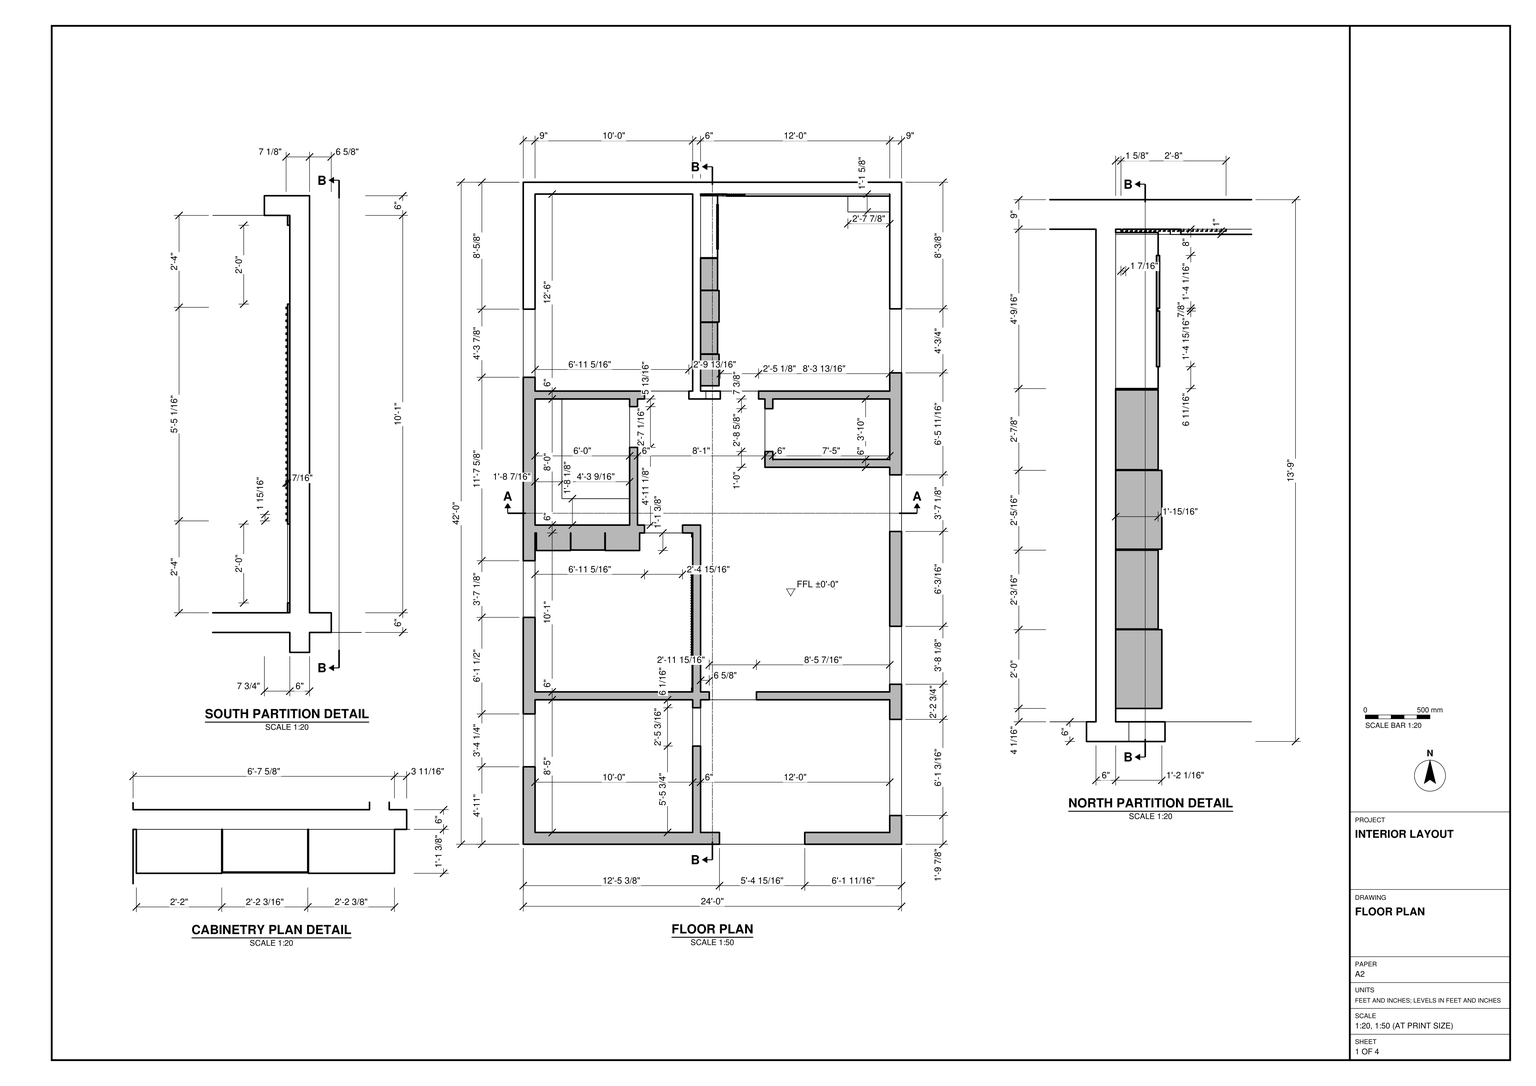
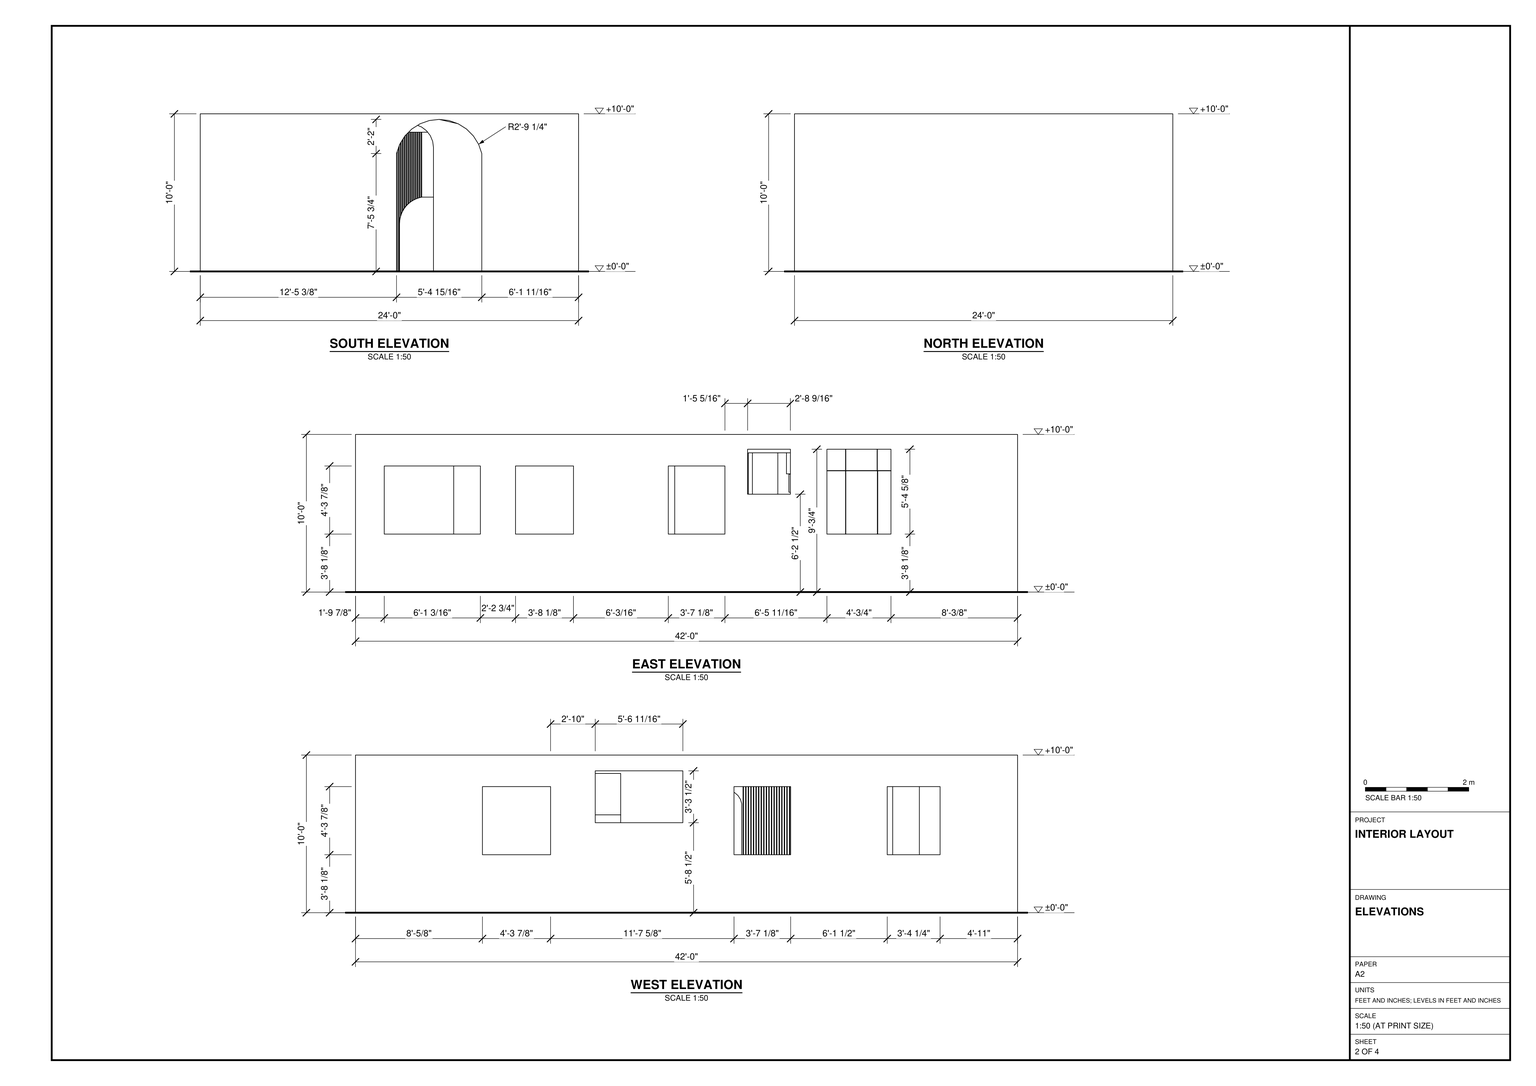
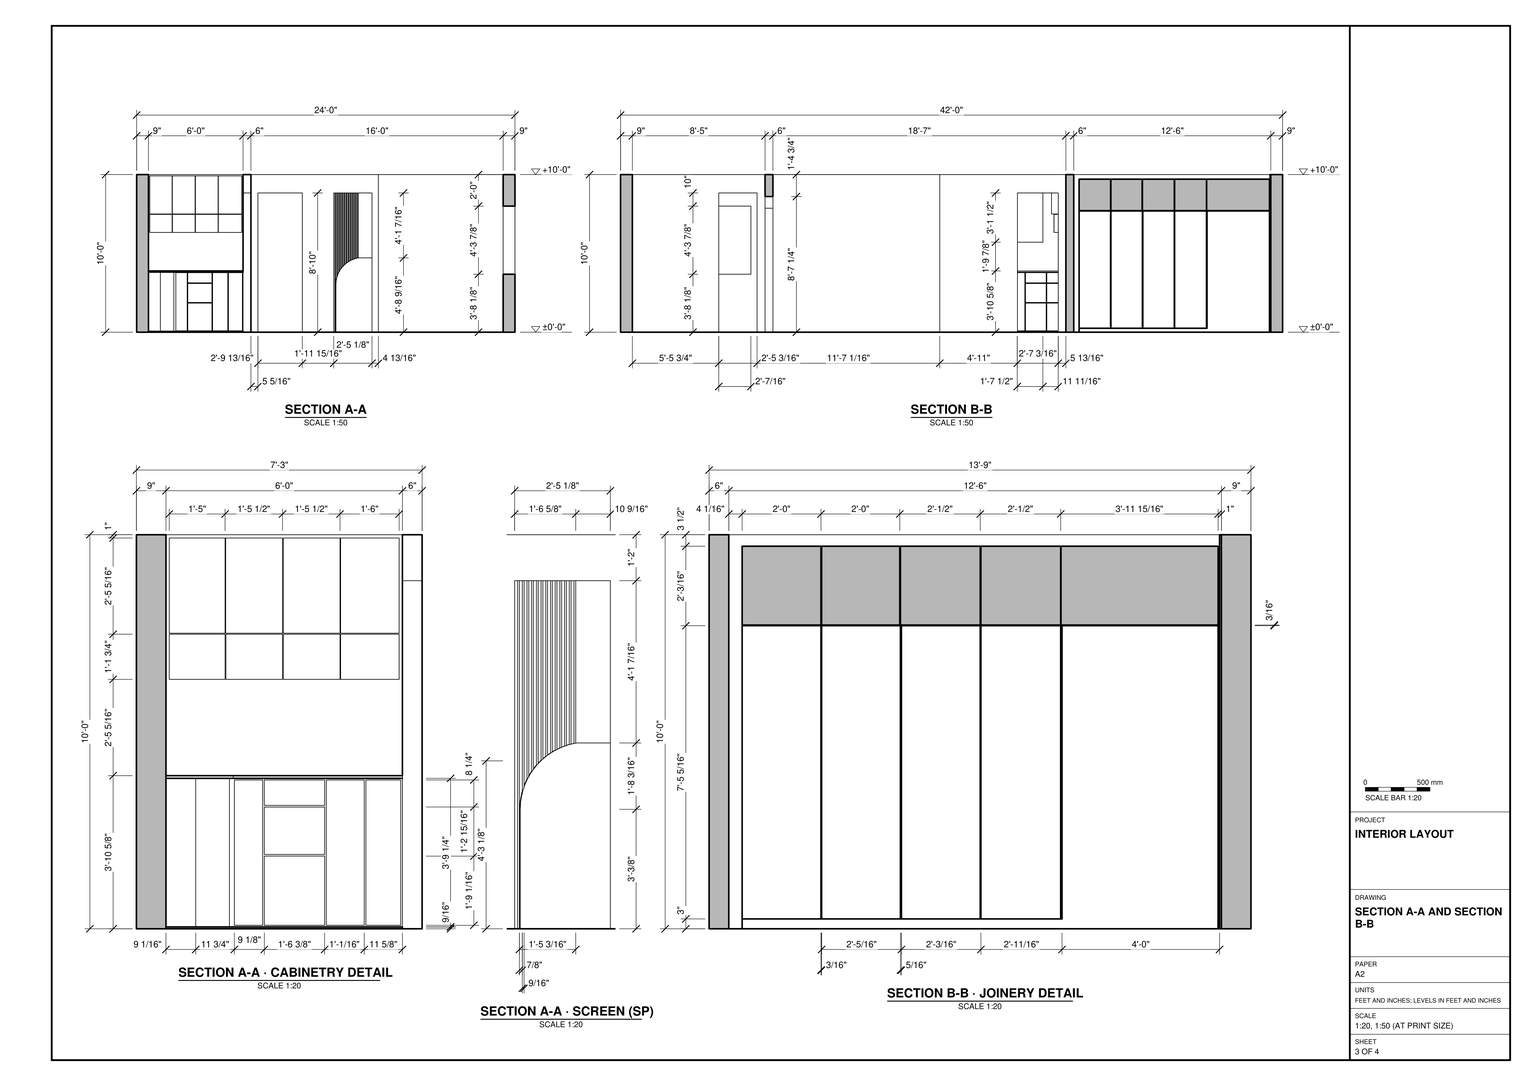
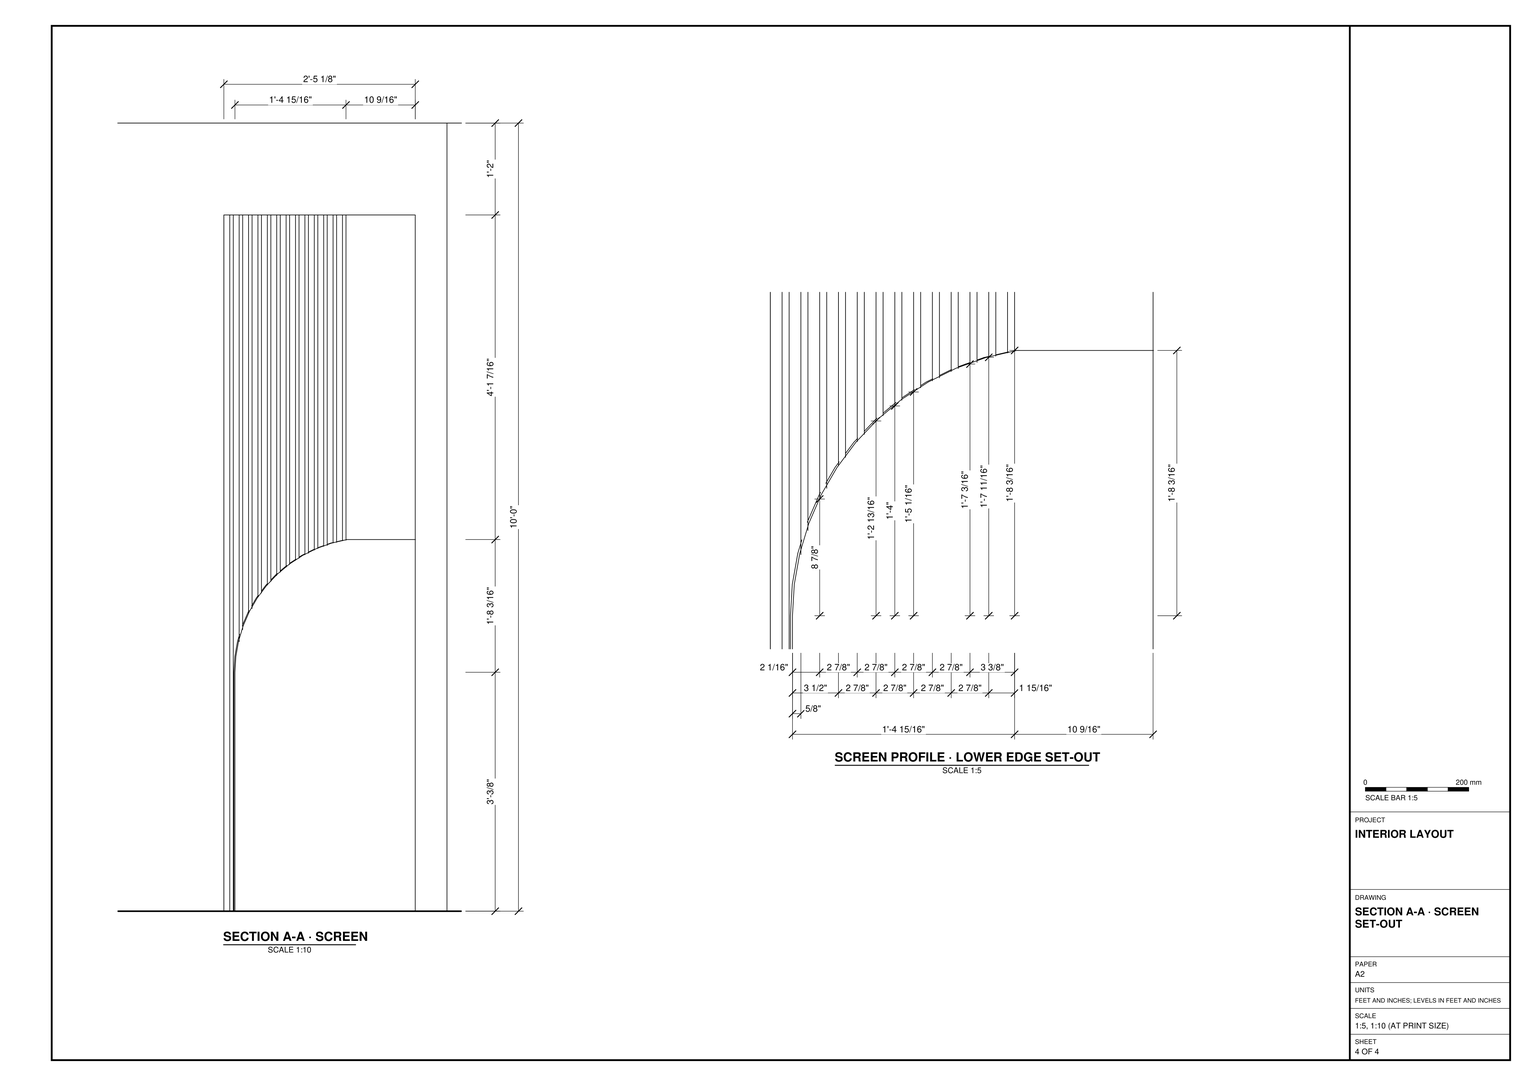
Build the interior in SketchUp from task_files/diagram_01.pdf. Work in feet and inches. Set the finished floor at ±0'-0" and model the rectangular shell 24'-0" wide, 42'-0" long and 10'-0" high. Use the floor plan to set out the 9" perimeter walls and 6" internal partitions. Follow the breaks in the partitions so the passages connect the end rooms with the central space as drawn.

Form the offset arched entrance in the south wall and leave the north wall solid. Use the east and west elevations to locate the window openings and set their individual sill and head heights. Model the fitted cabinetry in section A-A with its worktop, base storage, central drawers and upper cupboards. Include the separate three-bay cabinet run from the plan detail. Follow section B-B for the tall storage fronts and the overhead cupboards that continue above the clear bay. Build the screen with vertical slats terminating along the curved profile shown in section A-A.

Keep the floor, walls and each joinery or furniture piece in separate groups or components, and use components for repeated parts. Decor and loose items may be any suitable library components. Save one SketchUp model as output_files/interior_with_fitted_cabinetry_and_slatted_screen.skp.

# SketchUp Ruby script. Lengths in inches.
U = 1.inch
M = Sketchup.active_model
def pt(a) = Geom::Point3d.new(a.map { |v| v * U })
def face(e, loops, mat)
  f = e.add_face(loops[0].map { |a| pt(a) })
  loops[1..].each { |l| e.add_face(l.map { |a| pt(a) }).erase! }
  f.material = f.back_material = mat if mat
  f
end
# faces: each face lists its corners as indices into pts; further lists are holes
def faces(e, pts, list, mat = nil) = list.each { |f| face(e, (f[0].is_a?(Array) ? f : [f]).map { |l| l.map { |i| pts[i] } }, mat) }
# xy, xz, yz: faces in a plane at the given z, y or x. An outline is a flat list of corners, or four numbers for a rectangle; further outlines are holes
def ring(l) = l.size == 4 ? [[l[0], l[1]], [l[2], l[1]], [l[2], l[3]], [l[0], l[3]]] : l.each_slice(2).to_a
def flat(e, list, mat, &to3) = list.each { |f| face(e, (f[0].is_a?(Array) ? f : [f]).map { |l| ring(l).map { |u, v| to3.(u, v) } }, mat) }
def xy(e, z, list, mat = nil) = flat(e, list, mat) { |x, y| [x, y, z] }
def xz(e, y, list, mat = nil) = flat(e, list, mat) { |x, z| [x, y, z] }
def yz(e, x, list, mat = nil) = flat(e, list, mat) { |y, z| [x, y, z] }
def lines(e, pts, list) = list.each { |a, b| e.add_line(pt(pts[a]), pt(pts[b])) }
# prism: a flat outline (further loops are holes) pulled along v
def prism(e, loops, v, mat = nil)
  f = face(e, loops, mat); d = Geom::Vector3d.new(v.map { |x| x * U })
  f.pushpull(f.normal.samedirection?(d) ? d.length : -d.length)
end
def box(e, o, s, mat = nil) = prism(e, [[o, [o[0] + s[0], o[1], o[2]], [o[0] + s[0], o[1] + s[1], o[2]], [o[0], o[1] + s[1], o[2]]]], [0, 0, s[2]], mat)
def at(x, y, z, deg = 0) = Geom::Transformation.translation(pt([x, y, z])) * Geom::Transformation.rotation(ORIGIN, Z_AXIS, deg.degrees)
def axes(o, x, y, z) = Geom::Transformation.new([*x, 0, *y, 0, *z, 0, *pt(o).to_a, 1])
def part(name) = M.definitions.add(name)
# library, detail: a bought-in or finely detailed component or shape, given as its bounding box
def library(name, o, s) = part(name).tap { |d| box(d.entities, o, s) }
def detail(e, o, s) = box(e.add_group.entities, o, s)
def put(e, d, t, mat = nil) = e.add_instance(d, t).tap { |i| i.material = mat if mat }
def group(e, t, mat = nil) = e.add_group.tap { |g| g.transformation = t; g.material = mat if mat }.entities
root = M.entities
M.materials.add("[0027_PeachPuff]").color = [255, 218, 185]
M.materials.add("[0081_CadetBlue]").color = [95, 158, 160]
M.materials.add("[0095_LightBlue]").color = [173, 216, 230]
M.materials.add("[Carrera Marble]").color = [207, 207, 207]
M.materials.add("[Color C01]").color = [255, 229, 204]
M.materials.add("[Color M00]").color = [255, 255, 255]
M.materials.add("[Field Square Tile]").color = [217, 201, 169]
M.materials.add("[Field Square Tile]1").color = [217, 201, 169]
M.materials.add("[Tile Hexagon White]").color = [213, 206, 204]
M.materials.add("[Translucent Glass Gray]").color = [128, 128, 128]
M.materials["[Translucent Glass Gray]"].alpha = 0.5
M.materials.add("[Wallpaper Thin Brown Stripes]").color = [182, 160, 118]
c1 = library("Group\#10",[0,0,0],[72,96,45.25])
c2 = library("Group\#11",[0,-13.625,0],[144.15,13.625,120])
c3 = library("Group\#14",[-1.125,0,0],[1.125,121,120])
xy(root,0,[[0,0,149.39,0,149.39,9,135,9,135,74.75,129,74.75,129,9,9,9,9,110,129,110,129,103.9375,135,103.9375,135,110,141.625,110,141.625,116,135,116,135,243,121.25,243,121.25,237,129,237,129,116,9,116,9,237,10,237,10,223.625,88.6,223.625,88.6,237,92.3125,237,92.3125,243,87,243,87,302.125,81,302.125,81,243,9,243,9,339,81,339,81,333.1875,87,333.1875,87,339,92.32,339,92.32,345,9,345,9,495,129,495,129,345,126.12,345,126.12,339,150.03,339,150.03,345,135,345,135,493.4375,147.9375,493.4375,147.9375,493.98,135,493.98,135,495,279,495,279,493.4375,279.15,493.4375,279.15,345,179.17,345,179.17,339,184,339,184,331.625,190,331.625,190,339,279,339,279,293,190,293,190,299,184,299,184,287,279,287,279,116,177.53,116,177.53,110,279,110,279,9,214.32,9,214.32,0,288,0,288,504,0,504],[129,74.75,135,103.9375],[20.43,243,81,251.01],[279,345,279.15,493.4375],[147.9375,493.4375,279,493.4375,279,495,135,495,135,493.98,147.9375,493.98]])
xy(root,0,[[135,349.0625,147.9375,493.4375]],"[Color M00]")
xy(root,0.5625,[[9,243,9,339,28.33,339,28.33,261.8125,81,261.8125,81,243]])
xy(root,2,[[36,223.625,62.4,223.625,62.4,237,62.2,237,62.2,224,36.2,224,36.2,237,36,237]])
xy(root,3,[[135,349.0625,147.9375,373.0625],[147.9375,349.0625,149.0625,373.0625],[135,373.26,147.9375,397.26],[135,397.5625,147.9375,421.5625],[147.9375,397.5625,149.0625,421.5625],
  [135,421.76,147.9375,446.0625],[135,446.0625,147.9375,446.46],[135,493.98,147.9375,494]])
xy(root,3,[[135,421.5625,147.9375,421.76]],"[0081_CadetBlue]")
xy(root,3,[[135,373.0625,147.9375,373.26],[135,397.26,147.9375,397.5625]],"[0095_LightBlue]")
xy(root,10,[[147.4375,453.15,147.9375,453.15,147.9375,470.08,147.8125,470.08,147.8125,470.96,147.9375,470.96,147.9375,487,147.4375,487],[147.9375,453.15,148.375,470.08],[147.9375,470.96,148.375,487]])
xy(root,44.125,[[279,21.875,288,95.0625],[0,58.98,9,99.23],[279,121.8125,288,165.9375],[0,172.73,9,215.875],[279,238.11,288,281.22],
  [0,355.5,9,407.375],[279,358.875,288,407.625]])
xy(root,45.8125,[[9,243,9,339,29.45,339,29.45,263.12,81,263.12,81,243]])
xy(root,46.625,[[9,243,81,243,81,263.12,29.45,263.12,29.45,339,9,339]],"[Carrera Marble]")
xy(root,68.5,[[0,254.8125,9,321.5]])
xy(root,74.5,[[279,298.5,288,331.0625]])
xy(root,75.96,[[10,329.9375,27,339],[27.25,329.9375,44.5,339],[44.75,330,62,339],[62.1875,330,80,339]],"[Color C01]")
xy(root,81.8125,[[9,243,81,250.5]],"[Carrera Marble]")
xy(root,82.8125,[[44.0625,239.1875,54.25,250.5],[10,241.1875,18.75,250.5],[21,241.625,29.3125,250.5],[31.5,242.25,41.875,250.5],[69,244.1875,80,250.5]])
xy(root,82.8125,[[56.4375,244.375,66.8125,250.5]],"[Carrera Marble]")
xy(root,82.99,[[10,223.625,36,237],[62.4,223.625,88.6,237],[36.2,224,62.2,237]],"[0027_PeachPuff]")
xy(root,83.1875,[[10,223.625,36,237],[36.21,223.625,62.2,237],[62.4,223.625,88.4,237]])
xy(root,89.7,[[10,329.9375,27,339],[27.25,329.9375,44.5,339],[44.75,330,62,339],[62.1875,330,80,339]],"[Color C01]")
xy(root,90,[[10,328.0625,27,339],[27.1875,328.0625,44.5,339],[44.75,328.0625,62,339],[62.1875,328.0625,80,339]],"[Wallpaper Thin Brown Stripes]")
xy(root,92.3,[[135,421.76,147.9375,446.0625],[135,446.46,147.9375,494]])
xy(root,92.3,[[135,349.0625,149.0625,373.0625],[135,373.26,147.9375,397.26],[135,397.5625,149.0625,421.5625]],"[0081_CadetBlue]")
xy(root,92.5,[[135,349.0625,149.0625,373.0625],[135,373.26,149.0625,397.0625],[135,397.26,149.0625,421.5625],[135,421.76,149.0625,446.0625],[135,446.15,149.0625,494]])
xy(root,95.25,[[44.0625,239.1875,54.25,250.5],[10,241.1875,18.75,250.5],[21,241.625,29.3125,250.5],[31.5,242.25,41.875,250.5],[69,244.1875,80,250.5],
  [56.4375,244.375,66.8125,250.5]])
xy(root,96,[[279,21.875,288,95.0625],[0,58.98,9,99.23],[279,121.8125,288,165.9375],[0,172.73,9,215.875],[279,238.11,288,281.22],
  [0,355.5,9,407.375]])
xy(root,96.25,[[9,243,81,250.5]],"[Color C01]")
xy(root,96.4375,[[10,243,19.8,249.8125],[19.95,243,30.3125,249.8125],[30.5,243,42.8125,249.8125],[43,243,55.375,249.8125],[55.5,243,67.8125,249.8125],
  [68,243,80.75,249.8125]])
xy(root,106,[[129,74.75,135,103.9375],[92.3125,237,121.25,243],[184,299,190,331.625],[81,302.125,87,333.1875],[92.32,339,126.12,345]])
xy(root,106.01,[[150.03,339,179.17,345]])
xy(root,108,[[0,254.8125,9,321.5]])
xy(root,108.75,[[279,298.5,288,331.0625],[279,358.875,288,407.625]])
xy(root,116.5,[[135,349.0625,149.0625,373.0625],[135,373.26,149.0625,397.0625],[135,397.26,149.0625,421.5625],[135,421.76,149.0625,446.0625],[135,446.15,149.0625,494]],"[Carrera Marble]")
xy(root,119,[[10,243,19.8,249.8125],[19.95,243,30.3125,249.8125],[30.5,243,42.8125,249.8125],[43,243,55.375,249.8125],[55.5,243,67.8125,249.8125],
  [68,243,80.75,249.8125],[10,328.0625,27,339],[27.1875,328.0625,44.5,339],[44.75,328.0625,62,339],[62.1875,328.0625,80,339]],"[Wallpaper Thin Brown Stripes]")
xy(root,120,[[[0,0,288,504],[135,116,135,243,87,243,87,339,184,339,184,287,279,287,279,116],[135,345,279,495],[9,345,129,495],[135,9,279,110],[9,116,129,237],[9,9,129,110],[9,243,81,339],[190,293,279,339]]])
xy(root,120,[[10,223.625,36,237],[36.21,223.625,62.2,237],[62.4,223.625,88.4,237]],"[Carrera Marble]")
xz(root,0,[[0,0,149.39,0,149.39,89.75,151.83,96.8125,155.78,103.15,161.05,108.45,167.375,112.44,174.43,114.91,181.85,115.75,189.28,114.91,196.33,112.44,202.65,108.45,207.92,103.15,211.875,96.8125,214.32,89.75,214.32,0,288,0,288,120,0,120]])
xz(root,9,[[9,0,129,120],[135,0,135,120,279,120,279,0,214.32,0,214.32,89.75,211.875,96.8125,207.92,103.15,202.65,108.45,196.33,112.44,189.28,114.91,181.85,115.75,174.43,114.91,167.375,112.44,161.05,108.45,155.78,103.15,151.83,96.8125,149.39,89.75,149.39,0]])
xz(root,21.875,[[279,44.125,288,96]])
xz(root,58.98,[[0,44.125,9,96]])
xz(root,74.75,[[129,0,135,106]])
xz(root,95.0625,[[279,44.125,288,96]])
xz(root,99.23,[[0,44.125,9,96]])
xz(root,103.9375,[[129,0,135,106]])
xz(root,110,[[9,0,129,120],[135,0,141.625,0,141.625,94.375,142.24,99.02,144.03,103.35,146.88,107.07,150.6,109.92,154.93,111.72,159.58,112.33,164.23,111.72,168.56,109.92,172.28,107.07,175.13,103.35,176.92,99.02,177.53,94.375,177.53,0,279,0,279,120,135,120]])
xz(root,116,[[9,0,129,120],[135,0,135,120,279,120,279,0,177.53,0,177.53,94.375,176.92,99.02,175.13,103.35,172.28,107.07,168.56,109.92,164.23,111.72,159.58,112.33,154.93,111.72,150.6,109.92,146.88,107.07,144.03,103.35,142.24,99.02,141.625,94.375,141.625,0]])
xz(root,121.8125,[[279,44.125,288,96]])
xz(root,165.9375,[[279,44.125,288,96]])
xz(root,172.73,[[0,44.125,9,96]])
xz(root,215.875,[[0,44.125,9,96]])
xz(root,223.625,[[10,2,36,82.99],[62.4,2,88.6,82.99]],"[0027_PeachPuff]")
xz(root,223.625,[[10,0,88.6,2],[10,83.1875,36,120],[36.21,83.1875,62.2,120],[62.4,83.1875,88.4,120]],"[Carrera Marble]")
xz(root,224,[[36.2,2,62.2,82.99]],"[0027_PeachPuff]")
xz(root,237,[[9,0,10,0,10,82.99,36,82.99,36,2,36.2,2,36.2,82.99,62.2,82.99,62.2,2,62.4,2,62.4,82.99,88.6,82.99,88.6,0,92.3125,0,92.3125,106,121.25,106,121.25,0,129,0,129,120,88.4,120,88.4,83.1875,62.4,83.1875,62.4,120,62.2,120,62.2,83.1875,36.21,83.1875,36.21,120,36,120,36,83.1875,10,83.1875,10,120,9,120],[10,83.1875,36,120],[36.21,83.1875,62.2,120]])
xz(root,237,[[62.4,83.1875,88.4,120]],"[Carrera Marble]")
xz(root,238.11,[[279,44.125,288,96]])
xz(root,239.1875,[[44.0625,82.8125,54.25,95.25]])
xz(root,241.1875,[[10,82.8125,18.75,95.25]])
xz(root,241.625,[[21,82.8125,29.3125,95.25]])
xz(root,242.25,[[31.5,82.8125,41.875,95.25]])
xz(root,243,[[9,0,81,0.5625],[87,0,87,120,135,120,135,0,121.25,0,121.25,106,92.3125,106,92.3125,0],[9,0.5625,81,46.625],[9,46.625,81,81.8125],[[9,96.25,81,120],[68,96.4375,80.75,119],[43,96.4375,55.375,119],[55.5,96.4375,67.8125,119],[30.5,96.4375,42.8125,119],[19.95,96.4375,30.3125,119],[10,96.4375,19.8,119]]])
xz(root,244.1875,[[69,82.8125,80,95.25]])
xz(root,244.375,[[56.4375,82.8125,66.8125,95.25]],"[Carrera Marble]")
xz(root,249.8125,[[10,96.4375,19.8,119],[19.95,96.4375,30.3125,119],[30.5,96.4375,42.8125,119],[43,96.4375,55.375,119],[55.5,96.4375,67.8125,119],
  [68,96.4375,80.75,119]],"[Wallpaper Thin Brown Stripes]")
xz(root,250.5,[[[9,81.8125,19.75,96.25],[10,82.8125,18.75,95.25]],[[20,81.8125,30.3125,96.25],[21,82.8125,29.3125,95.25]],[[30.5,81.8125,42.875,96.25],[31.5,82.8125,41.875,95.25]],[[43.0625,81.8125,55.25,96.25],[44.0625,82.8125,54.25,95.25]],[[55.4375,81.8125,67.8125,96.25],[56.4375,82.8125,66.8125,95.25]],
  [[68,81.8125,81,96.25],[69,82.8125,80,95.25]]],"[Color C01]")
xz(root,250.5,[[19.75,81.8125,20,96.25],[30.3125,81.8125,30.5,96.25],[42.875,81.8125,43.0625,96.25],[55.25,81.8125,55.4375,96.25],[67.8125,81.8125,68,96.25],
  [10,82.8125,18.75,95.25],[21,82.8125,29.3125,95.25],[31.5,82.8125,41.875,95.25],[44.0625,82.8125,54.25,95.25],[56.4375,82.8125,66.8125,95.25],
  [69,82.8125,80,95.25]],"[Translucent Glass Gray]")
xz(root,254.8125,[[0,68.5,9,108]])
xz(root,263.12,[[29.45,45.8125,81,46.625]])
xz(root,281.22,[[279,44.125,288,96]])
xz(root,287,[[184,0,279,120]])
xz(root,293,[[190,0,279,120]])
xz(root,298.5,[[279,74.5,288,108.75]])
xz(root,299,[[184,0,190,106]])
xz(root,302.125,[[81,0,87,106]])
xz(root,321.5,[[0,68.5,9,108]])
xz(root,328.0625,[[10,90,27,119],[27.1875,90,44.5,119],[44.75,90,62,119],[62.1875,90,80,119]],"[Wallpaper Thin Brown Stripes]")
xz(root,329.9375,[[10,75.96,27,89.7],[27.25,75.96,44.5,89.7]],"[Color C01]")
xz(root,330,[[44.75,75.96,62,89.7],[62.1875,75.96,80,89.7]],"[Color C01]")
xz(root,331.0625,[[279,74.5,288,108.75]])
xz(root,331.625,[[184,0,190,106]])
xz(root,333.1875,[[81,0,87,106]])
xz(root,339,[[9,0,18.06,0.5625],[[18.06,0,81,0,81,120,9,120,9,46.625,29.45,46.625,29.45,45.8125,28.33,45.8125,28.33,0.5625,18.06,0.5625],[62.1875,90,80,119],[27.1875,90,44.5,119],[44.75,90,62,119],[10,90,27,119],[62.1875,75.96,80,89.7],[27.25,75.96,44.5,89.7],[44.75,75.96,62,89.7],[10,75.96,27,89.7]],[87,0,92.32,0,92.32,106,126.12,106,126.12,0,150.03,0,150.03,106.01,179.17,106.01,179.17,0,184,0,184,120,87,120],[190,0,279,120],[9,0.5625,18.06,45.8125],
  [18.06,0.5625,28.33,45.8125]])
xz(root,345,[[9,0,9,120,129,120,129,0,126.12,0,126.12,106,92.32,106,92.32,0],[135,0,135,120,279,120,279,0,179.17,0,179.17,106.01,150.03,106.01,150.03,0]])
xz(root,349.0625,[[135,0,147.9375,3],[135,92.5,149.0625,116.5]])
xz(root,349.0625,[[135,3,149.0625,92.3]],"[0081_CadetBlue]")
xz(root,355.5,[[0,44.125,9,96]])
xz(root,358.875,[[279,44.125,288,108.75]])
xz(root,373.0625,[[135,3,149.0625,92.3]],"[0081_CadetBlue]")
xz(root,373.0625,[[135,92.5,149.0625,116.5]],"[Carrera Marble]")
xz(root,373.26,[[135,92.5,149.0625,116.5]])
xz(root,373.26,[[135,3,147.9375,92.3]],"[0081_CadetBlue]")
xz(root,397.0625,[[135,92.5,149.0625,116.5]])
xz(root,397.26,[[135,3,147.9375,92.3]],"[0081_CadetBlue]")
xz(root,397.26,[[135,92.5,149.0625,116.5]],"[Carrera Marble]")
xz(root,397.5625,[[135,3,149.0625,92.3]],"[0081_CadetBlue]")
xz(root,407.375,[[0,44.125,9,96]])
xz(root,407.625,[[279,44.125,288,108.75]])
xz(root,421.5625,[[135,92.5,149.0625,116.5]])
xz(root,421.5625,[[135,3,149.0625,92.3]],"[0081_CadetBlue]")
xz(root,421.76,[[135,3,147.9375,92.3]],"[0081_CadetBlue]")
xz(root,421.76,[[135,92.5,149.0625,116.5]],"[Carrera Marble]")
xz(root,446.0625,[[135,92.5,149.0625,116.5]])
xz(root,446.0625,[[135,3,147.9375,92.3]],"[0081_CadetBlue]")
xz(root,446.15,[[135,92.5,149.0625,116.5]],"[Carrera Marble]")
xz(root,446.46,[[135,3,147.9375,92.3]],"[0095_LightBlue]")
xz(root,453.15,[[147.4375,10,147.9375,74.45]])
xz(root,453.15,[[147.9375,10,148.375,74.45]],"[Translucent Glass Gray]")
xz(root,470.08,[[147.8125,10,148.375,85.3]],"[Translucent Glass Gray]")
xz(root,470.96,[[147.8125,10,148.375,85.22]],"[Translucent Glass Gray]")
xz(root,487,[[147.4375,10,147.9375,74.45]])
xz(root,487,[[147.9375,10,148.375,74.45]],"[Translucent Glass Gray]")
xz(root,493.98,[[135,0,147.9375,3]])
xz(root,494,[[135,3,147.9375,92.3],[135,92.5,149.0625,116.5]])
xz(root,495,[[9,0,129,120]])
xz(root,504,[[0,0,288,120]])
yz(root,0,[[[0,0,504,120],[355.5,44.125,407.375,96],[254.8125,68.5,321.5,108],[172.73,44.125,215.875,96],[58.98,44.125,99.23,96]]])
yz(root,9,[[[9,0,110,120],[58.98,44.125,99.23,96]],[116,0,117,120],[[117,0,237,120],[172.73,44.125,215.875,96]],[243,0,339,45.8125],[[345,0,495,120],[355.5,44.125,407.375,96]],
  [243,45.8125,339,46.625],[[243,46.625,339,46.625,339,120,243,120,243,96.25,250.5,96.25,250.5,81.8125,243,81.8125],[254.8125,68.5,321.5,108]]])
yz(root,10,[[223.625,0,237,2],[223.625,2,237,82.99],[329.9375,75.96,339,89.7],[241.1875,82.8125,250.5,95.25],[223.625,83.1875,237,120]])
yz(root,10,[[328.0625,90,339,119],[243,96.4375,249.8125,119]],"[Wallpaper Thin Brown Stripes]")
yz(root,18.75,[[241.1875,82.8125,250.5,95.25]])
yz(root,19.8,[[243,96.4375,249.8125,119]],"[Wallpaper Thin Brown Stripes]")
yz(root,19.95,[[243,96.4375,249.8125,119]],"[Wallpaper Thin Brown Stripes]")
yz(root,21,[[241.625,82.8125,250.5,95.25]])
yz(root,27,[[329.9375,75.96,339,89.7]],"[Color C01]")
yz(root,27,[[328.0625,90,339,119]],"[Wallpaper Thin Brown Stripes]")
yz(root,27.1875,[[328.0625,90,339,119]],"[Wallpaper Thin Brown Stripes]")
yz(root,27.25,[[329.9375,75.96,339,89.7]])
yz(root,29.3125,[[241.625,82.8125,250.5,95.25]])
yz(root,29.45,[[263.12,45.8125,339,46.625]])
yz(root,30.3125,[[243,96.4375,249.8125,119]],"[Wallpaper Thin Brown Stripes]")
yz(root,30.5,[[243,96.4375,249.8125,119]],"[Wallpaper Thin Brown Stripes]")
yz(root,31.5,[[242.25,82.8125,250.5,95.25]])
yz(root,36,[[223.625,2,237,82.99]],"[0027_PeachPuff]")
yz(root,36,[[223.625,83.1875,237,120]],"[Carrera Marble]")
yz(root,36.2,[[224,2,237,82.99]],"[0027_PeachPuff]")
yz(root,36.21,[[223.625,83.1875,237,120]])
yz(root,41.875,[[242.25,82.8125,250.5,95.25]])
yz(root,42.8125,[[243,96.4375,249.8125,119]],"[Wallpaper Thin Brown Stripes]")
yz(root,43,[[243,96.4375,249.8125,119]],"[Wallpaper Thin Brown Stripes]")
yz(root,44.0625,[[239.1875,82.8125,250.5,95.25]])
yz(root,44.5,[[329.9375,75.96,339,89.7]],"[Color C01]")
yz(root,44.5,[[328.0625,90,339,119]],"[Wallpaper Thin Brown Stripes]")
yz(root,44.75,[[330,75.96,339,89.7]])
yz(root,44.75,[[328.0625,90,339,119]],"[Wallpaper Thin Brown Stripes]")
yz(root,54.25,[[239.1875,82.8125,250.5,95.25]])
yz(root,55.375,[[243,96.4375,249.8125,119]],"[Wallpaper Thin Brown Stripes]")
yz(root,55.5,[[243,96.4375,249.8125,119]],"[Wallpaper Thin Brown Stripes]")
yz(root,56.4375,[[244.375,82.8125,250.5,95.25]])
yz(root,62,[[330,75.96,339,89.7]],"[Color C01]")
yz(root,62,[[328.0625,90,339,119]],"[Wallpaper Thin Brown Stripes]")
yz(root,62.1875,[[330,75.96,339,89.7]])
yz(root,62.1875,[[328.0625,90,339,119]],"[Wallpaper Thin Brown Stripes]")
yz(root,62.2,[[224,2,237,82.99]],"[0027_PeachPuff]")
yz(root,62.2,[[223.625,83.1875,237,120]],"[Carrera Marble]")
yz(root,62.4,[[223.625,83.1875,237,120]])
yz(root,62.4,[[223.625,2,237,82.99]],"[0027_PeachPuff]")
yz(root,66.8125,[[244.375,82.8125,250.5,95.25]],"[Carrera Marble]")
yz(root,67.8125,[[243,96.4375,249.8125,119]],"[Wallpaper Thin Brown Stripes]")
yz(root,68,[[243,96.4375,249.8125,119]],"[Wallpaper Thin Brown Stripes]")
yz(root,69,[[244.1875,82.8125,250.5,95.25]])
yz(root,80,[[244.1875,82.8125,250.5,95.25]])
yz(root,80,[[330,75.96,339,89.7]],"[Color C01]")
yz(root,80,[[328.0625,90,339,119]],"[Wallpaper Thin Brown Stripes]")
yz(root,80.75,[[243,96.4375,249.8125,119]])
yz(root,81,[[251.01,0,251.01,0.5625,261.8125,0.5625,261.8125,45.8125,263.12,45.8125,263.12,46.625,243,46.625,243,81.8125,250.5,81.8125,250.5,96.25,243,96.25,243,120,339,120,339,0,333.1875,0,333.1875,106,302.125,106,302.125,0]])
yz(root,87,[[243,0,302.125,0,302.125,106,333.1875,106,333.1875,0,339,0,339,120,243,120]])
yz(root,88.4,[[223.625,83.1875,237,120]],"[Carrera Marble]")
yz(root,88.6,[[223.625,0,237,2]])
yz(root,88.6,[[223.625,2,237,82.99]],"[0027_PeachPuff]")
yz(root,92.3125,[[237,0,243,106]])
yz(root,92.32,[[339,0,345,106]])
yz(root,121.25,[[237,0,243,106]])
yz(root,126.12,[[339,0,345,106]])
yz(root,129,[[9,0,9,120,110,120,110,0,103.9375,0,103.9375,106,74.75,106,74.75,0],[345,0,495,120]])
yz(root,135,[[9,0,74.75,0,74.75,106,103.9375,106,103.9375,0,110,0,110,120,9,120],[116,0,243,120],[[345,0,349.0625,0,349.0625,92.3,373.0625,92.3,373.0625,3,373.26,3,373.26,92.3,397.26,92.3,397.26,3,397.5625,3,397.5625,92.3,421.5625,92.3,421.5625,3,421.76,3,421.76,92.3,446.0625,92.3,446.0625,3,446.46,3,446.46,92.3,494,92.3,494,3,493.98,3,493.98,0,495,0,495,120,345,120],[446.15,92.5,494,116.5],[397.26,92.5,421.5625,116.5],[421.76,92.5,446.0625,116.5],[349.0625,92.5,373.0625,116.5],[373.26,92.5,397.0625,116.5]],[349.0625,3,373.0625,92.3],[373.26,3,397.26,92.3],
  [397.5625,3,421.5625,92.3],[421.76,3,446.0625,92.3]])
yz(root,141.625,[[110,0,116,94.375]])
yz(root,147.4375,[[453.15,10,487,10,487,74.45,485.23,77.5,482.91,80.17,480.13,82.35,476.99,83.97,473.59,84.96,470.08,85.3,466.56,84.96,463.16,83.97,460.02,82.35,457.24,80.17,454.92,77.5,453.15,74.45]])
yz(root,147.8125,[[470.08,10,470.96,10,470.96,85.22,470.08,85.3]],"[Translucent Glass Gray]")
yz(root,147.9375,[[470.96,85.22,470.96,85.3,470.08,85.3]])
yz(root,147.9375,[[373.26,3,397.26,92.3],[421.76,3,446.0625,92.3]],"[0081_CadetBlue]")
yz(root,147.9375,[[349.0625,0,493.98,3],[[446.46,3,494,92.3],[453.15,10,453.15,74.45,454.92,77.5,457.24,80.17,460.02,82.35,463.16,83.97,466.56,84.96,470.08,85.3,470.96,85.3,470.96,85.22,473.59,84.96,476.99,83.97,480.13,82.35,482.91,80.17,485.23,77.5,487,74.45,487,10]]],"[0095_LightBlue]")
yz(root,148.375,[[453.15,10,470.08,10,470.08,85.3,466.56,84.96,463.16,83.97,460.02,82.35,457.24,80.17,454.92,77.5,453.15,74.45],[470.96,10,487,10,487,74.45,485.23,77.5,482.91,80.17,480.13,82.35,476.99,83.97,473.59,84.96,470.96,85.22]],"[Translucent Glass Gray]")
yz(root,149.0625,[[349.0625,3,373.0625,92.3],[397.5625,3,421.5625,92.3]],"[0081_CadetBlue]")
yz(root,149.0625,[[349.0625,92.5,373.0625,116.5],[373.26,92.5,397.0625,116.5],[397.26,92.5,421.5625,116.5],[421.76,92.5,446.0625,116.5],[446.15,92.5,494,116.5]],"[Carrera Marble]")
yz(root,149.39,[[0,0,9,89.75]])
yz(root,150.03,[[339,0,345,106.01]])
yz(root,177.53,[[110,0,116,94.375]])
yz(root,179.17,[[339,0,345,106.01]])
yz(root,184,[[287,0,287,120,339,120,339,0,331.625,0,331.625,106,299,106,299,0]])
yz(root,190,[[293,0,299,0,299,106,331.625,106,331.625,0,339,0,339,120,293,120]])
yz(root,214.32,[[0,0,9,89.75]])
yz(root,279,[[[9,0,110,120],[21.875,44.125,95.0625,96]],[[116,0,287,120],[121.8125,44.125,165.9375,96],[238.11,44.125,281.22,96]],[[293,0,339,120],[298.5,74.5,331.0625,108.75]],[[345,0,495,120],[358.875,44.125,407.625,108.75]]])
yz(root,288,[[[0,0,504,120],[21.875,44.125,95.0625,96],[358.875,44.125,407.625,108.75],[121.8125,44.125,165.9375,96],[238.11,44.125,281.22,96],[298.5,74.5,331.0625,108.75]]])
p = [[147.9375,454.92,77.5],[147.9375,453.15,74.45],[147.4375,453.15,74.45],[147.4375,454.92,77.5],[148.375,453.15,74.45],[148.375,454.92,77.5],
  [147.9375,487,74.45],[147.9375,485.23,77.5],[147.4375,485.23,77.5],[147.4375,487,74.45],[148.375,485.23,77.5],[148.375,487,74.45],
  [147.9375,457.24,80.17],[147.4375,457.24,80.17],[148.375,457.24,80.17],[147.9375,482.91,80.17],[147.4375,482.91,80.17],[148.375,482.91,80.17],
  [147.9375,460.02,82.35],[147.4375,460.02,82.35],[148.375,460.02,82.35],[147.9375,480.13,82.35],[147.4375,480.13,82.35],[148.375,480.13,82.35],
  [147.9375,463.16,83.97],[147.4375,463.16,83.97],[148.375,463.16,83.97],[147.9375,476.99,83.97],[147.4375,476.99,83.97],[148.375,476.99,83.97],
  [147.9375,466.56,84.96],[147.4375,466.56,84.96],[148.375,466.56,84.96],[147.9375,473.59,84.96],[147.4375,473.59,84.96],[148.375,473.59,84.96],
  [147.9375,470.08,85.3],[147.4375,470.08,85.3],[147.8125,470.08,85.3],[148.375,470.08,85.3],[147.9375,470.96,85.22],[147.8125,470.96,85.22],
  [148.375,470.96,85.22],[151.83,0,96.8125],[149.39,0,89.75],[149.39,9,89.75],[151.83,9,96.8125],[214.32,0,89.75],
  [211.875,0,96.8125],[211.875,9,96.8125],[214.32,9,89.75],[141.625,116,94.375],[142.24,116,99.02],[142.24,110,99.02],
  [141.625,110,94.375],[176.92,116,99.02],[177.53,116,94.375],[177.53,110,94.375],[176.92,110,99.02],[155.78,0,103.15],
  [155.78,9,103.15],[207.92,0,103.15],[207.92,9,103.15],[144.03,116,103.35],[144.03,110,103.35],[175.13,116,103.35],
  [175.13,110,103.35],[161.05,0,108.45],[161.05,9,108.45],[202.65,0,108.45],[202.65,9,108.45],[146.88,116,107.07],
  [146.88,110,107.07],[172.28,116,107.07],[172.28,110,107.07],[150.6,116,109.92],[150.6,110,109.92],[168.56,116,109.92],
  [168.56,110,109.92],[167.375,0,112.44],[167.375,9,112.44],[196.33,0,112.44],[196.33,9,112.44],[154.93,116,111.72],
  [154.93,110,111.72],[164.23,116,111.72],[164.23,110,111.72],[159.58,116,112.33],[159.58,110,112.33],[174.43,0,114.91],
  [174.43,9,114.91],[189.28,0,114.91],[189.28,9,114.91],[181.85,0,115.75],[181.85,9,115.75]]
faces(root,p,[[0,1,2,3],[6,7,8,9],[12,0,3,13],[7,15,16,8],[18,12,13,19],[15,21,22,16],[24,18,19,25],[21,27,28,22],
  [30,24,25,31],[27,33,34,28],[36,30,31,37,38],[33,40,41,38,37,34],[40,36,38,41],[43,44,45,46],[47,48,49,50],[51,52,53,54],
  [55,56,57,58],[59,43,46,60],[48,61,62,49],[52,63,64,53],[65,55,58,66],[67,59,60,68],[61,69,70,62],[63,71,72,64],
  [73,65,66,74],[71,75,76,72],[77,73,74,78],[79,67,68,80],[69,81,82,70],[75,83,84,76],[85,77,78,86],[83,87,88,84],
  [87,85,86,88],[89,79,80,90],[81,91,92,82],[93,89,90,94],[91,93,94,92]])
faces(root,p,[[0,1,4,5],[6,7,10,11],[12,0,5,14],[7,15,17,10],[18,12,14,20],[15,21,23,17],[24,18,20,26],[21,27,29,23],
  [30,24,26,32],[27,33,35,29],[36,30,32,39],[33,40,42,35]],"[Translucent Glass Gray]")
g1 = group(root,at(9,9,0))
xy(g1,0,[[0,0,120,101]])
g2 = group(root,at(9,116,0),"[Field Square Tile]")
xy(g2,0,[[0,0,120,121]])
g3 = group(root,at(9,243,0),"[Carrera Marble]")
xy(g3,0,[[0,0,72,96]],"[Tile Hexagon White]")
g4 = group(root,at(9,345,0))
xy(g4,0,[[0,0,120,150]])
g5 = group(root,at(135,345,0),"[Color M00]")
xy(g5,0,[[0,0,144,150]],"[Field Square Tile]1")
g6 = group(root,at(184,293,0))
xy(g6,0,[[6,0,95,0,95,46,6,46,6,38.625,0,38.625,0,6,6,6]])
g7 = group(root,at(135,0,0))
xy(g7,0,[[14.39,0,79.32,0,79.32,9,144,9,144,110,0,110,0,9,14.39,9]])
g8 = group(root,at(81,110,0))
xy(g8,0,[[60.625,0,96.53,0,96.53,6,198,6,198,177,103,177,103,229,98.17,229,98.17,235,58.03,235,58.03,229,45.12,229,45.12,235,11.32,235,11.32,229,6,229,6,223.1875,0,223.1875,0,192.125,6,192.125,6,133,11.3125,133,11.3125,127,40.25,127,40.25,133,54,133,54,6,60.625,6]])
g9 = group(root,at(9,243,0))
xy(g9,0,[[17.81,8.01,17.81,17.7,17.87,17.7,17.87,17.76,72,17.76,72,8.01],[17.81,17.7,17.87,96]])
xy(g9,0.5625,[[0,0,72,0,72,17.76,17.87,17.76,17.87,96,0,96]])
xz(g9,17.76,[[17.87,0,72,0.5625]])
xz(g9,96,[[17.81,0,17.87,0.5625]])
yz(g9,17.87,[[17.76,0,96,0.5625]])
yz(g9,72,[[8.01,0,17.76,0.5625]])
p = [[11.43,8.01,0],[17.81,8.01,0]]
lines(g9,p,[[0,1]])
put(root,c1,at(9,243,0.5625))
put(root,c2,at(135,495,0))
put(root,c3,at(129,116,0))
